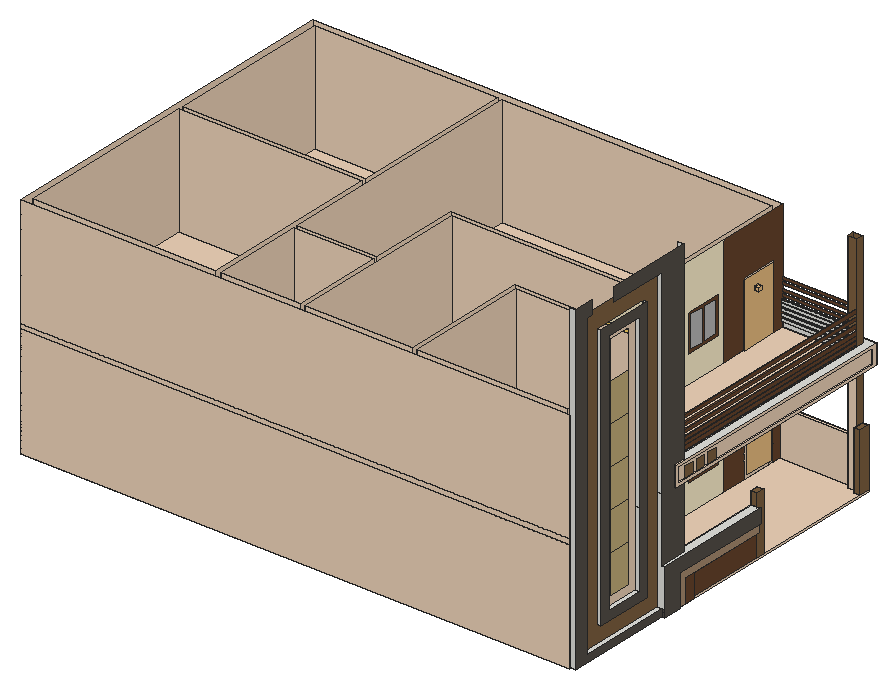
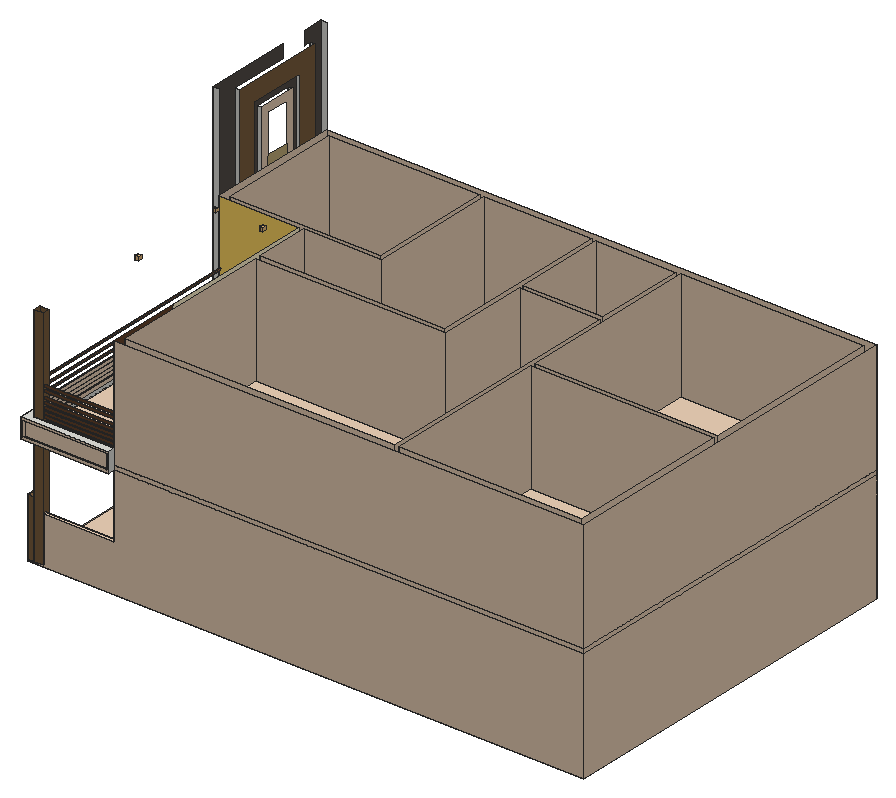
# SketchUp Ruby script. Lengths in inches.
U = 1.inch
M = Sketchup.active_model
def pt(a) = Geom::Point3d.new(a.map { |v| v * U })
def face(e, loops, mat)
  f = e.add_face(loops[0].map { |a| pt(a) })
  loops[1..].each { |l| e.add_face(l.map { |a| pt(a) }).erase! }
  f.material = f.back_material = mat if mat
  f
end
# faces: each face lists its corners as indices into pts; further lists are holes
def faces(e, pts, list, mat = nil) = list.each { |f| face(e, (f[0].is_a?(Array) ? f : [f]).map { |l| l.map { |i| pts[i] } }, mat) }
# xy, xz, yz: faces in a plane at the given z, y or x. An outline is a flat list of corners, or four numbers for a rectangle; further outlines are holes
def ring(l) = l.size == 4 ? [[l[0], l[1]], [l[2], l[1]], [l[2], l[3]], [l[0], l[3]]] : l.each_slice(2).to_a
def flat(e, list, mat, &to3) = list.each { |f| face(e, (f[0].is_a?(Array) ? f : [f]).map { |l| ring(l).map { |u, v| to3.(u, v) } }, mat) }
def xy(e, z, list, mat = nil) = flat(e, list, mat) { |x, y| [x, y, z] }
def xz(e, y, list, mat = nil) = flat(e, list, mat) { |x, z| [x, y, z] }
def yz(e, x, list, mat = nil) = flat(e, list, mat) { |y, z| [x, y, z] }
def lines(e, pts, list) = list.each { |a, b| e.add_line(pt(pts[a]), pt(pts[b])) }
# prism: a flat outline (further loops are holes) pulled along v
def prism(e, loops, v, mat = nil)
  f = face(e, loops, mat); d = Geom::Vector3d.new(v.map { |x| x * U })
  f.pushpull(f.normal.samedirection?(d) ? d.length : -d.length)
end
def box(e, o, s, mat = nil) = prism(e, [[o, [o[0] + s[0], o[1], o[2]], [o[0] + s[0], o[1] + s[1], o[2]], [o[0], o[1] + s[1], o[2]]]], [0, 0, s[2]], mat)
def at(x, y, z, deg = 0) = Geom::Transformation.translation(pt([x, y, z])) * Geom::Transformation.rotation(ORIGIN, Z_AXIS, deg.degrees)
def axes(o, x, y, z) = Geom::Transformation.new([*x, 0, *y, 0, *z, 0, *pt(o).to_a, 1])
def part(name) = M.definitions.add(name)
# library, detail: a bought-in or finely detailed component or shape, given as its bounding box
def library(name, o, s) = part(name).tap { |d| box(d.entities, o, s) }
def detail(e, o, s) = box(e.add_group.entities, o, s)
def put(e, d, t, mat = nil) = e.add_instance(d, t).tap { |i| i.material = mat if mat }
def group(e, t, mat = nil) = e.add_group.tap { |g| g.transformation = t; g.material = mat if mat }.entities
root = M.entities
M.materials.add("D01_Frost_White").color = [255, 242, 206]
M.materials.add("D03_Lemon_Mist").color = [255, 216, 101]
M.materials.add("Glass_Mirror_01").color = [185, 185, 185]
M.materials.add("Metal_10_1K").color = [196, 175, 123]
M.materials.add("Plywood_01_1K").color = [125, 96, 64]
M.materials.add("Roofing_01_1K").color = [84, 79, 73]
M.materials.add("ThomThom - Beard1").color = [168, 140, 112]
M.materials.add("ThomThom - Complexion1").color = [237, 210, 184]
M.materials.add("Wood_Veneer_15_1K").color = [103, 69, 45]
c1 = library("porta+4",[0.2,-5.42,1.33],[46.55,4.72,83.21])
c2 = library("Sphere Light\#6",[-3.83,-3.83,-3.83],[7.66,7.66,7.66])
c3 = library("Sphere Light\#7",[-3.85,-3.85,-3.85],[7.7,7.7,7.7])
c4 = library("Sphere Light\#8",[-4.15,-4.15,-4.15],[8.3,8.3,8.3])
c5 = library("Sphere Light\#9",[-3.2,-3.2,-3.2],[6.4,6.4,6.4])
c6 = library("Sphere Light\#10",[-3.49,-3.49,-3.49],[6.98,6.98,6.98])
c7 = library("Sphere Light\#11",[-4,-4,-4],[8,8,8])
c8 = library("Sphere Light\#2",[-2.48,-2.48,-2.48],[4.96,4.96,4.96])
c9 = library("Sphere Light\#1",[-2.41,-2.41,-2.41],[4.82,4.82,4.82])
c10 = library("Sphere Light",[-2.11,-2.11,-2.11],[4.22,4.22,4.22])
xy(root,2,[[720,0,720,297.66,728,297.66,728,190.54,730,190.54,730,165,732,165,732,141,728,141,728,0],[9,9,249,249],[255,9,360,129],[366,9,507,9,507,177,609,177,609,249,366,249],[513,9,711,171],
  [9,255,249,471],[719.19,297.66,728,308.57],[720,466.42,728,480]])
xy(root,2,[[708,471,720,480]],"ThomThom - Complexion1")
xy(root,11,[[722,18,728,141]])
xy(root,32,[[728,190.54,730,297.66]],"ThomThom - Beard1")
xy(root,35,[[722,42,728,117]])
xy(root,41,[[609,351.03,615,371.03]])
xy(root,44,[[730,165,732,297.66]],"Roofing_01_1K")
xy(root,47,[[722,54,728,105]])
xy(root,62,[[728,141,732,141,732,297.66,720,297.66,720,177,728,177]])
xy(root,78.34,[[719.19,297.66,728,308.57],[720,466.42,728,480]],"Plywood_01_1K")
xy(root,83,[[609,351.03,615,371.03]])
xy(root,146,[[720,177,720,480.02,615,480.02,615,489,731,489,731,177]])
xy(root,146,[[728,160.5,731,177]],"ThomThom - Complexion1")
xy(root,149,[[728,163.5,731,177],[728,177,731,483],[618,486,728,489]],"ThomThom - Complexion1")
xy(root,162.23,[[615,477.3125,708,479.11]])
xy(root,162.34,[[716.76,177,718.93,471]],"ThomThom - Complexion1")
xy(root,165.75,[[615,477.3125,708,479.11]],"Wood_Veneer_15_1K")
xy(root,166.14,[[716.76,177,718.93,471]],"Wood_Veneer_15_1K")
xy(root,167.64,[[615,477.3125,708,479.11]])
xy(root,168.53,[[716.76,177,718.93,471]],"ThomThom - Complexion1")
xy(root,169.07,[[728,163.5,731,177],[728,177,731,483],[618,486,728,489]],"ThomThom - Complexion1")
xy(root,171.16,[[615,477.3125,708,479.11]],"Wood_Veneer_15_1K")
xy(root,172.07,[[720,177,731,177,731,489,615,489,615,480.02,720,480.02]])
xy(root,172.07,[[728,160.5,731,177]],"ThomThom - Complexion1")
xy(root,172.33,[[716.76,177,718.93,471]],"Wood_Veneer_15_1K")
xy(root,173.54,[[716.76,177,718.93,471]],"ThomThom - Complexion1")
xy(root,174.29,[[615,477.3125,708,479.11]])
xy(root,177.34,[[716.76,177,718.93,471]],"Wood_Veneer_15_1K")
xy(root,177.81,[[615,477.3125,708,479.11]],"Wood_Veneer_15_1K")
xy(root,178.69,[[716.76,177,718.93,471]],"ThomThom - Complexion1")
xy(root,179.57,[[615,477.3125,708,479.11]])
xy(root,182.5,[[716.76,177,718.93,471]],"Wood_Veneer_15_1K")
xy(root,183.09,[[615,477.3125,708,479.11]],"Wood_Veneer_15_1K")
xy(root,184.3125,[[716.76,177,718.93,471]],"ThomThom - Complexion1")
xy(root,184.75,[[594.11,477.3125,708,479.11]])
xy(root,188.12,[[716.76,177,718.93,471]],"Wood_Veneer_15_1K")
xy(root,188.27,[[594.11,477.3125,708,479.11]],"Wood_Veneer_15_1K")
xy(root,193,[[609,351.03,615,371.03]])
xy(root,196.33,[[716.76,177,718.93,471]],"Wood_Veneer_15_1K")
xy(root,204.68,[[716.76,177,718.93,471]],"Wood_Veneer_15_1K")
xy(root,214,[[716.76,177,718.93,471]],"Wood_Veneer_15_1K")
xy(root,235,[[609,351.03,615,371.03]])
xz(root,0,[[720,2,728,424]])
xz(root,18,[[722,11,728,406]])
xz(root,42,[[722,35,728,382]])
xz(root,54,[[722,47,728,370]])
xz(root,105,[[722,47,728,146],[722,146,728,370]])
xz(root,117,[[722,35,728,146],[722,146,728,382]])
xz(root,141,[[722,11,732,11,732,62,728,62,728,146,722,146],[722,146,728,406]])
xz(root,141,[[728,2,732,7.79],[728,7.79,732,11]],"Roofing_01_1K")
xz(root,160.5,[[728,146,731,172.07]],"ThomThom - Complexion1")
xz(root,163.5,[[728,149,731,169.07]],"ThomThom - Complexion1")
xz(root,165,[[730,2,732,32],[730,32,732,44]],"Roofing_01_1K")
xz(root,177,[[720,62,728,146],[720,172.07,728,424]])
xz(root,177,[[716.76,162.34,718.93,166.14],[716.76,168.53,718.93,172.33],[716.76,173.54,718.93,177.34],[716.76,178.69,718.93,182.5],[716.76,184.3125,718.93,188.12]],"ThomThom - Complexion1")
xz(root,190.54,[[728,2,730,32]],"Wood_Veneer_15_1K")
xz(root,297.66,[[719.19,2,720,78.34],[720,2,728,62],[728,32,728,62,732,62,732,44,730,44,730,32]])
xz(root,297.66,[[720,62,728,78.34]],"Plywood_01_1K")
xz(root,308.57,[[719.19,2,728,78.34]],"Plywood_01_1K")
xz(root,351.03,[[609,41,615,83],[609,193,615,235]])
xz(root,371.03,[[609,41,615,83],[609,193,615,235]])
xz(root,466.42,[[720,2,728,78.34]],"Plywood_01_1K")
xz(root,471,[[708,190,720,298]],"Plywood_01_1K")
xz(root,471,[[[708,2,720,190],[716.76,184.3125,718.93,188.12],[716.76,178.69,718.93,182.5],[716.76,173.54,718.93,177.34],[716.76,168.53,718.93,172.33],[716.76,162.34,718.93,166.14]]],"ThomThom - Complexion1")
xz(root,477.3125,[[615,162.23,708,165.75],[615,167.64,708,171.16],[615,174.29,708,177.81],[615,179.57,708,183.09],[594.11,184.75,708,188.27]])
xz(root,479.11,[[615,162.23,708,165.75],[615,167.64,708,171.16],[615,174.29,708,177.81],[615,179.57,708,183.09],[594.11,184.75,708,188.27],
  [594.11,191,708,194.52],[594.11,196.75,708,200.27],[594.11,204.61,708,208.13],[594.11,210.66,708,214.18]],"Wood_Veneer_15_1K")
xz(root,480,[[708,2,720,298],[720,2,728,78.34]],"Plywood_01_1K")
xz(root,480.02,[[615,146,720,172.07]])
xz(root,483,[[728,149,731,169.07]],"ThomThom - Complexion1")
xz(root,486,[[618,149,728,169.07]],"ThomThom - Complexion1")
xz(root,489,[[[615,146,731,172.07],[618,149,728,169.07]]],"ThomThom - Complexion1")
yz(root,594.11,[[477.3125,184.75,479.11,188.27]])
yz(root,609,[[351.03,41,371.03,83],[351.03,193,371.03,235]])
yz(root,615,[[480.02,146,489,172.07],[477.3125,162.23,479.11,165.75],[477.3125,167.64,479.11,171.16],[477.3125,174.29,479.11,177.81],[477.3125,179.57,479.11,183.09]])
yz(root,618,[[486,149,489,169.07]],"ThomThom - Complexion1")
yz(root,708,[[477.3125,162.23,479.11,165.75],[477.3125,167.64,479.11,171.16],[477.3125,174.29,479.11,177.81],[477.3125,179.57,479.11,183.09],[477.3125,184.75,479.11,188.27]])
yz(root,708,[[471,2,480,298]],"Plywood_01_1K")
yz(root,716.76,[[177,162.34,471,166.14],[177,168.53,471,172.33],[177,173.54,471,177.34],[177,178.69,471,182.5],[177,184.3125,471,188.12]],"ThomThom - Complexion1")
yz(root,718.93,[[177,162.34,471,166.14],[177,168.53,471,172.33],[177,173.54,471,177.34],[177,178.69,471,182.5],[177,184.3125,471,188.12],
  [177,192.52,471,196.33],[177,200.875,471,204.68],[177,210.2,471,214]],"Wood_Veneer_15_1K")
yz(root,719.19,[[297.66,2,308.57,78.34]])
yz(root,720,[[177,2,297.66,62],[466.42,2,480,78.34],[177,146,480.02,172.07]])
yz(root,720,[[471,2,480,62],[471,62,480,65],[471,65,480,298]],"Plywood_01_1K")
yz(root,722,[[64,57,95,107.5],[64,107.5,95,158],[64,158,95,208.5],[64,208.5,95,259],[64,259,95,309.5]],"Metal_10_1K")
yz(root,722,[[[18,11,141,406],[42,35,117,382]]],"Plywood_01_1K")
yz(root,722,[[[54,47,105,370],[64,57,95,360]]],"ThomThom - Complexion1")
yz(root,728,[[297.66,2,308.57,78.34],[466.42,2,480,78.34]],"Plywood_01_1K")
yz(root,728,[[0,2,141,2,141,11,18,11,18,406,27.04,406,27.04,424,0,424],[[42,35,117,382],[54,47,105,370]],[141,62,177,62,177,146,160.5,146,160.5,172.07,177,172.07,177,424,63.32,424,63.32,406,141,406]],"Roofing_01_1K")
yz(root,728,[[163.5,149,483,169.07],[486,149,489,169.07]],"ThomThom - Complexion1")
yz(root,728,[[190.54,2,297.66,32]],"Wood_Veneer_15_1K")
yz(root,730,[[165,2,177,2,177,32,297.66,32,297.66,44,165,44]],"ThomThom - Beard1")
yz(root,730,[[177,2,190.54,32]],"Wood_Veneer_15_1K")
yz(root,731,[[[160.5,146,489,172.07],[163.5,149,483,169.07]]],"ThomThom - Complexion1")
yz(root,732,[[141,2,165,2,165,44,297.66,44,297.66,62,141,62]],"Roofing_01_1K")
yz(root,733.2,[[173.05,153.16,185.15,166.64],[191.37,153.16,203.46,166.64],[210.77,153.16,222.86,166.64]],"Plywood_01_1K")
p = [[255,471,2],[255,135,2],[360,135,2],[360,255,2],[711,177,146],[720,177,146],
  [615,249,146],[615,255,146],[609,249,146],[609,255,146],[615,255,2],[708,480,154],
  [708,480,173.37],[615,480,190],[615,480,173.37],[615,480,154],[708,480,190],[720,471,190],
  [708,471,190],[615,374.03,190],[615,326.03,190],[615,326.03,238],[615,374.03,238],[615,329.03,235],
  [615,329.03,193],[615,349.03,193],[615,351.03,235],[615,349.03,235],[615,351.03,193],[615,351.03,83],
  [615,349.03,83],[615,349.03,41],[615,351.03,41],[615,329.03,83],[615,326.03,86],[615,374.03,86],
  [615,326.03,38],[615,374.03,38],[615,329.03,41],[615,384,154],[615,384,298]]
lines(root,p,[[0,1],[2,1],[3,2],[4,5],[6,7],[8,9],[10,3],[11,12],[13,14],[15,11],[12,16],[14,15],
  [17,18],[19,20],[20,21],[21,22],[22,19],[23,24],[24,25],[26,27],[25,28],[27,25],[27,23],[29,30],
  [31,32],[30,31],[30,33],[34,35],[36,34],[37,36],[35,37],[33,38],[38,31],[39,40]])
g1 = group(root,at(0,0,0),"ThomThom - Complexion1")
xy(g1,0,[[0,0,0,480,728,480,728,177,720,177,720,0]])
xy(g1,2,[[255,135,360,135,360,255,609,255,609,471,255,471],[615,177,728,177,728,480,708,480,708,475.5,615,475.5],[609,255,615,471]])
xy(g1,5,[[609,420,615,462]])
xy(g1,62,[[615,475.5,708,480]])
xy(g1,83,[[609,420,615,462]])
xy(g1,146,[[[0,0,720,0,720,177,615,177,615,480,0,480],[366,9,366,249,609,249,609,255,360,255,360,135,255,135,255,471,609,471,609,177,507,177,507,9],[9,9,249,249],[9,255,249,471],[513,9,711,171],[255,9,360,129]]])
xz(g1,0,[[0,0,720,146]])
xz(g1,9,[[9,2,249,146],[255,2,360,146],[366,2,507,146],[513,2,609,146],[609,2,615,146],
  [615,2,711,146]])
xz(g1,129,[[255,2,360,146]])
xz(g1,135,[[255,2,360,146]])
xz(g1,171,[[513,2,609,146],[609,2,615,146],[615,2,711,146]])
xz(g1,177,[[720,0,728,0.27],[720,0.27,728,2],[507,2,609,146],[711,2,720,146]])
xz(g1,177,[[615,2,711,146]],"D03_Lemon_Mist")
xz(g1,249,[[9,2,249,146],[366,2,507,146],[507,2,513,146],[513,2,609,146]])
xz(g1,255,[[9,2,249,146],[360,2,609,146]])
xz(g1,420,[[609,5,615,83]])
xz(g1,462,[[609,5,615,83]])
xz(g1,471,[[9,2,249,146],[255,2,609,146]])
xz(g1,475.5,[[615,2,708,62]])
xz(g1,480,[[0,0,0,146,615,146,615,62,708,62,708,2,728,2,728,0]])
yz(g1,0,[[0,0,480,146]])
yz(g1,9,[[9,2,249,146],[255,2,471,146]])
yz(g1,249,[[9,2,249,146],[255,2,471,146]])
yz(g1,255,[[9,2,129,146],[135,2,471,146]])
yz(g1,360,[[9,2,129,146],[135,2,255,146]])
yz(g1,366,[[9,2,249,146]])
yz(g1,507,[[9,2,177,146]])
yz(g1,513,[[9,2,171,146]])
yz(g1,609,[[177,2,249,146],[[255,2,471,146],[420,5,462,83]]])
yz(g1,615,[[[417,2,465,86],[420,5,462,83]]])
yz(g1,615,[[[177,2,384,146],[326.03,38,374.03,86]]],"D01_Frost_White")
yz(g1,615,[[329.03,41,349.03,83],[351.03,41,371.03,83]],"Glass_Mirror_01")
yz(g1,615,[[384,2,417,2,417,86,465,86,465,2,475.5,2,475.5,62,480,62,480,146,384,146],[[326.03,38,374.03,86],[329.03,41,349.03,83],[351.03,41,371.03,83]]],"Wood_Veneer_15_1K")
yz(g1,708,[[475.5,2,480,62]])
yz(g1,711,[[9,2,171,146]])
yz(g1,720,[[0,0,177,146]])
yz(g1,728,[[177,0,480,2]])
p = [[615,471,146],[609,471,146]]
lines(g1,p,[[0,1]])
put(root,c1,axes([615.67,419.82,3.71],[0,0.88392,0],[0.96185,0,0],[0,0,0.93792]))
g2 = group(root,at(0,0,146),"ThomThom - Complexion1")
xy(g2,0,[[[0,0,720,480],[644.14,197.97,645.18,198.04,646.17,198.37,647.04,198.95,647.73,199.73,648.2,200.66,648.4,201.6875,648.34,202.73,648.01,203.72,647.43,204.59,646.65,205.28,645.72,205.75,644.69,205.96,643.65,205.89,642.66,205.56,641.79,204.98,641.1,204.2,640.63,203.27,640.42,202.24,640.49,201.2,640.82,200.21,641.4,199.34,642.18,198.65,643.11,198.18],[644.14,318,645.18,318.06,646.17,318.39,647.04,318.97,647.73,319.75,648.2,320.68,648.4,321.71,648.34,322.75,648.01,323.74,647.43,324.61,646.65,325.3,645.72,325.77,644.69,325.98,643.65,325.91,642.66,325.58,641.79,325,641.1,324.22,640.63,323.29,640.42,322.26,640.49,321.22,640.82,320.23,641.4,319.36,642.18,318.67,643.11,318.2],[695.98,318,697.02,318.06,698.01,318.39,698.88,318.97,699.57,319.75,700.04,320.68,700.25,321.71,700.18,322.75,699.85,323.74,699.28,324.61,698.49,325.3,697.56,325.77,696.54,325.98,695.49,325.91,694.5,325.58,693.63,325,692.94,324.22,692.47,323.29,692.27,322.26,692.33,321.22,692.66,320.23,693.24,319.36,694.02,318.67,694.95,318.2],[644.14,443.65,645.18,443.71,646.17,444.04,647.04,444.62,647.73,445.4,648.2,446.33,648.4,447.36,648.34,448.4,648.01,449.39,647.43,450.26,646.65,450.95,645.72,451.42,644.69,451.63,643.65,451.5625,642.66,451.23,641.79,450.66,641.1,449.875,640.63,448.9375,640.42,447.92,640.49,446.875,640.82,445.88,641.4,445.01,642.18,444.32,643.11,443.86],[695.98,443.65,697.02,443.71,698.01,444.04,698.88,444.62,699.57,445.4,700.04,446.33,700.25,447.36,700.18,448.4,699.85,449.39,699.28,450.26,698.49,450.95,697.56,451.42,696.54,451.63,695.49,451.5625,694.5,451.23,693.63,450.66,692.94,449.875,692.47,448.9375,692.27,447.92,692.33,446.875,692.66,445.88,693.24,445.01,694.02,444.32,694.95,443.86],[695.98,197.97,697.02,198.04,698.01,198.37,698.88,198.95,699.57,199.73,700.04,200.66,700.25,201.6875,700.18,202.73,699.85,203.72,699.28,204.59,698.49,205.28,697.56,205.75,696.54,205.96,695.49,205.89,694.5,205.56,693.63,204.98,692.94,204.2,692.47,203.27,692.27,202.24,692.33,201.2,692.66,200.21,693.24,199.34,694.02,198.65,694.95,198.18]]])
xy(g2,2,[[644.14,197.97,643.11,198.18,642.18,198.65,641.4,199.34,640.82,200.21,640.49,201.2,640.42,202.24,640.63,203.27,641.1,204.2,641.79,204.98,642.66,205.56,643.65,205.89,644.69,205.96,645.72,205.75,646.65,205.28,647.43,204.59,648.01,203.72,648.34,202.73,648.4,201.6875,648.2,200.66,647.73,199.73,647.04,198.95,646.17,198.37,645.18,198.04],[695.98,197.97,694.95,198.18,694.02,198.65,693.24,199.34,692.66,200.21,692.33,201.2,692.27,202.24,692.47,203.27,692.94,204.2,693.63,204.98,694.5,205.56,695.49,205.89,696.54,205.96,697.56,205.75,698.49,205.28,699.28,204.59,699.85,203.72,700.18,202.73,700.25,201.6875,700.04,200.66,699.57,199.73,698.88,198.95,698.01,198.37,697.02,198.04],[644.14,318,643.11,318.2,642.18,318.67,641.4,319.36,640.82,320.23,640.49,321.22,640.42,322.26,640.63,323.29,641.1,324.22,641.79,325,642.66,325.58,643.65,325.91,644.69,325.98,645.72,325.77,646.65,325.3,647.43,324.61,648.01,323.74,648.34,322.75,648.4,321.71,648.2,320.68,647.73,319.75,647.04,318.97,646.17,318.39,645.18,318.06],[695.98,318,694.95,318.2,694.02,318.67,693.24,319.36,692.66,320.23,692.33,321.22,692.27,322.26,692.47,323.29,692.94,324.22,693.63,325,694.5,325.58,695.49,325.91,696.54,325.98,697.56,325.77,698.49,325.3,699.28,324.61,699.85,323.74,700.18,322.75,700.25,321.71,700.04,320.68,699.57,319.75,698.88,318.97,698.01,318.39,697.02,318.06],[644.14,443.65,643.11,443.86,642.18,444.32,641.4,445.01,640.82,445.88,640.49,446.875,640.42,447.92,640.63,448.9375,641.1,449.875,641.79,450.66,642.66,451.23,643.65,451.5625,644.69,451.63,645.72,451.42,646.65,450.95,647.43,450.26,648.01,449.39,648.34,448.4,648.4,447.36,648.2,446.33,647.73,445.4,647.04,444.62,646.17,444.04,645.18,443.71],
  [695.98,443.65,694.95,443.86,694.02,444.32,693.24,445.01,692.66,445.88,692.33,446.875,692.27,447.92,692.47,448.9375,692.94,449.875,693.63,450.66,694.5,451.23,695.49,451.5625,696.54,451.63,697.56,451.42,698.49,450.95,699.28,450.26,699.85,449.39,700.18,448.4,700.25,447.36,700.04,446.33,699.57,445.4,698.88,444.62,698.01,444.04,697.02,443.71]])
xy(g2,6,[[0,0,720,480]])
xz(g2,0,[[0,0,720,6]])
xz(g2,480,[[0,0,720,6]])
yz(g2,0,[[0,0,480,6]])
yz(g2,720,[[0,0,480,6]])
p = [[644.14,197.97,0],[643.11,198.18,0],[643.11,198.18,2],[644.14,197.97,2],[645.18,198.04,0],[645.18,198.04,2],
  [646.17,198.37,0],[646.17,198.37,2],[695.98,197.97,0],[694.95,198.18,0],[694.95,198.18,2],[695.98,197.97,2],
  [697.02,198.04,0],[697.02,198.04,2],[698.01,198.37,0],[698.01,198.37,2],[642.18,198.65,0],[642.18,198.65,2],
  [694.02,198.65,0],[694.02,198.65,2],[647.04,198.95,0],[647.04,198.95,2],[698.88,198.95,0],[698.88,198.95,2],
  [641.4,199.34,0],[641.4,199.34,2],[693.24,199.34,0],[693.24,199.34,2],[647.73,199.73,0],[647.73,199.73,2],
  [699.57,199.73,0],[699.57,199.73,2],[640.82,200.21,0],[640.82,200.21,2],[692.66,200.21,0],[692.66,200.21,2],
  [648.2,200.66,0],[648.2,200.66,2],[700.04,200.66,0],[700.04,200.66,2],[640.49,201.2,0],[640.49,201.2,2],
  [692.33,201.2,0],[692.33,201.2,2],[648.4,201.6875,0],[648.4,201.6875,2],[700.25,201.6875,0],[700.25,201.6875,2],
  [640.42,202.24,0],[640.42,202.24,2],[692.27,202.24,0],[692.27,202.24,2],[648.34,202.73,0],[648.34,202.73,2],
  [700.18,202.73,0],[700.18,202.73,2],[640.63,203.27,0],[640.63,203.27,2],[692.47,203.27,0],[692.47,203.27,2],
  [648.01,203.72,0],[648.01,203.72,2],[699.85,203.72,0],[699.85,203.72,2],[641.1,204.2,0],[641.1,204.2,2],
  [692.94,204.2,0],[692.94,204.2,2],[647.43,204.59,0],[647.43,204.59,2],[699.28,204.59,0],[699.28,204.59,2],
  [641.79,204.98,0],[641.79,204.98,2],[693.63,204.98,0],[693.63,204.98,2],[646.65,205.28,0],[646.65,205.28,2],
  [698.49,205.28,0],[698.49,205.28,2],[642.66,205.56,0],[642.66,205.56,2],[694.5,205.56,0],[694.5,205.56,2],
  [645.72,205.75,0],[645.72,205.75,2],[697.56,205.75,0],[697.56,205.75,2],[643.65,205.89,0],[643.65,205.89,2],
  [695.49,205.89,0],[695.49,205.89,2],[644.69,205.96,0],[644.69,205.96,2],[696.54,205.96,0],[696.54,205.96,2],
  [644.14,318,0],[643.11,318.2,0],[643.11,318.2,2],[644.14,318,2],[645.18,318.06,0],[645.18,318.06,2],
  [695.98,318,0],[694.95,318.2,0],[694.95,318.2,2],[695.98,318,2],[697.02,318.06,0],[697.02,318.06,2],
  [646.17,318.39,0],[646.17,318.39,2],[698.01,318.39,0],[698.01,318.39,2],[642.18,318.67,0],[642.18,318.67,2],
  [694.02,318.67,0],[694.02,318.67,2],[647.04,318.97,0],[647.04,318.97,2],[698.88,318.97,0],[698.88,318.97,2],
  [641.4,319.36,0],[641.4,319.36,2],[693.24,319.36,0],[693.24,319.36,2],[647.73,319.75,0],[647.73,319.75,2],
  [699.57,319.75,0],[699.57,319.75,2],[640.82,320.23,0],[640.82,320.23,2],[692.66,320.23,0],[692.66,320.23,2],
  [648.2,320.68,0],[648.2,320.68,2],[700.04,320.68,0],[700.04,320.68,2],[640.49,321.22,0],[640.49,321.22,2],
  [692.33,321.22,0],[692.33,321.22,2],[648.4,321.71,0],[648.4,321.71,2],[700.25,321.71,0],[700.25,321.71,2],
  [640.42,322.26,0],[640.42,322.26,2],[692.27,322.26,0],[692.27,322.26,2],[648.34,322.75,0],[648.34,322.75,2],
  [700.18,322.75,0],[700.18,322.75,2],[640.63,323.29,0],[640.63,323.29,2],[692.47,323.29,0],[692.47,323.29,2],
  [648.01,323.74,0],[648.01,323.74,2],[699.85,323.74,0],[699.85,323.74,2],[641.1,324.22,0],[641.1,324.22,2],
  [692.94,324.22,0],[692.94,324.22,2],[647.43,324.61,0],[647.43,324.61,2],[699.28,324.61,0],[699.28,324.61,2],
  [641.79,325,0],[641.79,325,2],[693.63,325,0],[693.63,325,2],[646.65,325.3,0],[646.65,325.3,2],
  [698.49,325.3,0],[698.49,325.3,2],[642.66,325.58,0],[642.66,325.58,2],[694.5,325.58,0],[694.5,325.58,2],
  [645.72,325.77,0],[645.72,325.77,2],[697.56,325.77,0],[697.56,325.77,2],[643.65,325.91,0],[643.65,325.91,2],
  [695.49,325.91,0],[695.49,325.91,2],[644.69,325.98,0],[644.69,325.98,2],[696.54,325.98,0],[696.54,325.98,2],
  [644.14,443.65,0],[643.11,443.86,0],[643.11,443.86,2],[644.14,443.65,2],[645.18,443.71,0],[645.18,443.71,2],
  [695.98,443.65,0],[694.95,443.86,0],[694.95,443.86,2],[695.98,443.65,2],[697.02,443.71,0],[697.02,443.71,2],
  [646.17,444.04,0],[646.17,444.04,2],[698.01,444.04,0],[698.01,444.04,2],[642.18,444.32,0],[642.18,444.32,2],
  [694.02,444.32,0],[694.02,444.32,2],[647.04,444.62,0],[647.04,444.62,2],[698.88,444.62,0],[698.88,444.62,2],
  [641.4,445.01,0],[641.4,445.01,2],[693.24,445.01,0],[693.24,445.01,2],[647.73,445.4,0],[647.73,445.4,2],
  [699.57,445.4,0],[699.57,445.4,2],[640.82,445.88,0],[640.82,445.88,2],[692.66,445.88,0],[692.66,445.88,2],
  [648.2,446.33,0],[648.2,446.33,2],[700.04,446.33,0],[700.04,446.33,2],[640.49,446.875,0],[640.49,446.875,2],
  [692.33,446.875,0],[692.33,446.875,2],[648.4,447.36,0],[648.4,447.36,2],[700.25,447.36,0],[700.25,447.36,2],
  [640.42,447.92,0],[640.42,447.92,2],[692.27,447.92,0],[692.27,447.92,2],[648.34,448.4,0],[648.34,448.4,2],
  [700.18,448.4,0],[700.18,448.4,2],[640.63,448.9375,0],[640.63,448.9375,2],[692.47,448.9375,0],[692.47,448.9375,2],
  [648.01,449.39,0],[648.01,449.39,2],[699.85,449.39,0],[699.85,449.39,2],[641.1,449.875,0],[641.1,449.875,2],
  [692.94,449.875,0],[692.94,449.875,2],[647.43,450.26,0],[647.43,450.26,2],[699.28,450.26,0],[699.28,450.26,2],
  [641.79,450.66,0],[641.79,450.66,2],[693.63,450.66,0],[693.63,450.66,2],[646.65,450.95,0],[646.65,450.95,2],
  [698.49,450.95,0],[698.49,450.95,2],[642.66,451.23,0],[642.66,451.23,2],[694.5,451.23,0],[694.5,451.23,2],
  [645.72,451.42,0],[645.72,451.42,2],[697.56,451.42,0],[697.56,451.42,2],[643.65,451.5625,0],[643.65,451.5625,2],
  [695.49,451.5625,0],[695.49,451.5625,2],[644.69,451.63,0],[644.69,451.63,2],[696.54,451.63,0],[696.54,451.63,2]]
faces(g2,p,[[0,1,2,3],[4,0,3,5],[6,4,5,7],[8,9,10,11],[12,8,11,13],[14,12,13,15],[1,16,17,2],[9,18,19,10],
  [20,6,7,21],[22,14,15,23],[16,24,25,17],[18,26,27,19],[28,20,21,29],[30,22,23,31],[24,32,33,25],[26,34,35,27],
  [36,28,29,37],[38,30,31,39],[32,40,41,33],[34,42,43,35],[44,36,37,45],[46,38,39,47],[40,48,49,41],[42,50,51,43],
  [52,44,45,53],[54,46,47,55],[48,56,57,49],[50,58,59,51],[60,52,53,61],[62,54,55,63],[56,64,65,57],[58,66,67,59],
  [68,60,61,69],[70,62,63,71],[64,72,73,65],[66,74,75,67],[76,68,69,77],[78,70,71,79],[72,80,81,73],[74,82,83,75],
  [84,76,77,85],[86,78,79,87],[80,88,89,81],[82,90,91,83],[92,84,85,93],[94,86,87,95],[88,92,93,89],[90,94,95,91],
  [96,97,98,99],[100,96,99,101],[102,103,104,105],[106,102,105,107],[108,100,101,109],[110,106,107,111],[97,112,113,98],[103,114,115,104],
  [116,108,109,117],[118,110,111,119],[112,120,121,113],[114,122,123,115],[124,116,117,125],[126,118,119,127],[120,128,129,121],[122,130,131,123],
  [132,124,125,133],[134,126,127,135],[128,136,137,129],[130,138,139,131],[140,132,133,141],[142,134,135,143],[136,144,145,137],[138,146,147,139],
  [148,140,141,149],[150,142,143,151],[144,152,153,145],[146,154,155,147],[156,148,149,157],[158,150,151,159],[152,160,161,153],[154,162,163,155],
  [164,156,157,165],[166,158,159,167],[160,168,169,161],[162,170,171,163],[172,164,165,173],[174,166,167,175],[168,176,177,169],[170,178,179,171],
  [180,172,173,181],[182,174,175,183],[176,184,185,177],[178,186,187,179],[188,180,181,189],[190,182,183,191],[184,188,189,185],[186,190,191,187],
  [192,193,194,195],[196,192,195,197],[198,199,200,201],[202,198,201,203],[204,196,197,205],[206,202,203,207],[193,208,209,194],[199,210,211,200],
  [212,204,205,213],[214,206,207,215],[208,216,217,209],[210,218,219,211],[220,212,213,221],[222,214,215,223],[216,224,225,217],[218,226,227,219],
  [228,220,221,229],[230,222,223,231],[224,232,233,225],[226,234,235,227],[236,228,229,237],[238,230,231,239],[232,240,241,233],[234,242,243,235],
  [244,236,237,245],[246,238,239,247],[240,248,249,241],[242,250,251,243],[252,244,245,253],[254,246,247,255],[248,256,257,249],[250,258,259,251],
  [260,252,253,261],[262,254,255,263],[256,264,265,257],[258,266,267,259],[268,260,261,269],[270,262,263,271],[264,272,273,265],[266,274,275,267],
  [276,268,269,277],[278,270,271,279],[272,280,281,273],[274,282,283,275],[284,276,277,285],[286,278,279,287],[280,284,285,281],[282,286,287,283]])
put(g2,c2,at(695.96,201.95,2))
put(g2,c3,at(644.34,202.07,2))
put(g2,c4,at(644.54,321.85,2))
put(g2,c5,at(696.27,322.11,2))
put(g2,c6,at(696.66,446.875,2))
put(g2,c7,at(644.41,447.64,2))
g3 = group(root,at(0,0,152),"ThomThom - Complexion1")
xy(g3,0,[[0,0,720,480]])
xy(g3,2,[[9,9,249,249],[255,9,360,129],[366,9,507,9,507,177,609,177,609,249,366,249],[513,9,711,171],[255,135,360,135,360,255,609,255,609,471,255,471],
  [615,177,720,480],[9,255,249,471],[609,255,615,471]])
xy(g3,5,[[609,420,615,462]])
xy(g3,83,[[609,420,615,462]])
xz(g3,0,[[0,0,720,146]])
xz(g3,9,[[9,2,249,146],[255,2,360,146],[366,2,507,146],[513,2,711,146]])
xz(g3,129,[[255,2,360,146]])
xz(g3,135,[[255,2,360,146]])
xz(g3,171,[[513,2,711,146]])
xz(g3,177,[[507,2,609,146]])
xz(g3,177,[[615,2,720,146]],"D03_Lemon_Mist")
xz(g3,249,[[9,2,249,146],[366,2,609,146]])
xz(g3,255,[[9,2,249,146],[360,2,609,146]])
xz(g3,420,[[609,5,615,83]])
xz(g3,462,[[609,5,615,83]])
xz(g3,471,[[9,2,249,146],[255,2,609,146]])
xz(g3,480,[[0,0,0,146,615,146,615,2,720,2,720,0]])
yz(g3,0,[[0,0,480,146]])
yz(g3,9,[[9,2,249,146],[255,2,471,146]])
yz(g3,249,[[9,2,249,146],[255,2,471,146]])
yz(g3,255,[[9,2,129,146],[135,2,471,146]])
yz(g3,360,[[9,2,129,146],[135,2,255,146]])
yz(g3,366,[[9,2,249,146]])
yz(g3,507,[[9,2,177,146]])
yz(g3,513,[[9,2,171,146]])
yz(g3,609,[[177,2,249,146],[[255,2,471,146],[420,5,462,83]]])
yz(g3,615,[[[417,2,465,86],[420,5,462,83]]])
yz(g3,615,[[[177,2,384,146],[326.03,38,374.03,86]]],"D01_Frost_White")
yz(g3,615,[[329.03,41,349.03,83],[351.03,41,371.03,83]],"Glass_Mirror_01")
yz(g3,615,[[384,2,417,2,417,86,465,86,465,2,480,2,480,146,384,146],[[326.03,38,374.03,86],[329.03,41,349.03,83],[351.03,41,371.03,83]]],"Wood_Veneer_15_1K")
yz(g3,711,[[9,2,171,146]])
yz(g3,720,[[0,0,480,0,480,2,177,2,177,146,0,146]])
p = [[609,249,146],[609,255,146],[615,471,146],[609,471,146]]
lines(g3,p,[[0,1],[2,3]])
put(root,c1,at(610.72,416.8,152.66,90))
put(root,c8,at(705.19,328.4,298),"ThomThom - Complexion1")
put(root,c9,at(643.24,201.45,298),"ThomThom - Complexion1")
put(root,c10,at(705.19,201.45,298),"ThomThom - Complexion1")
